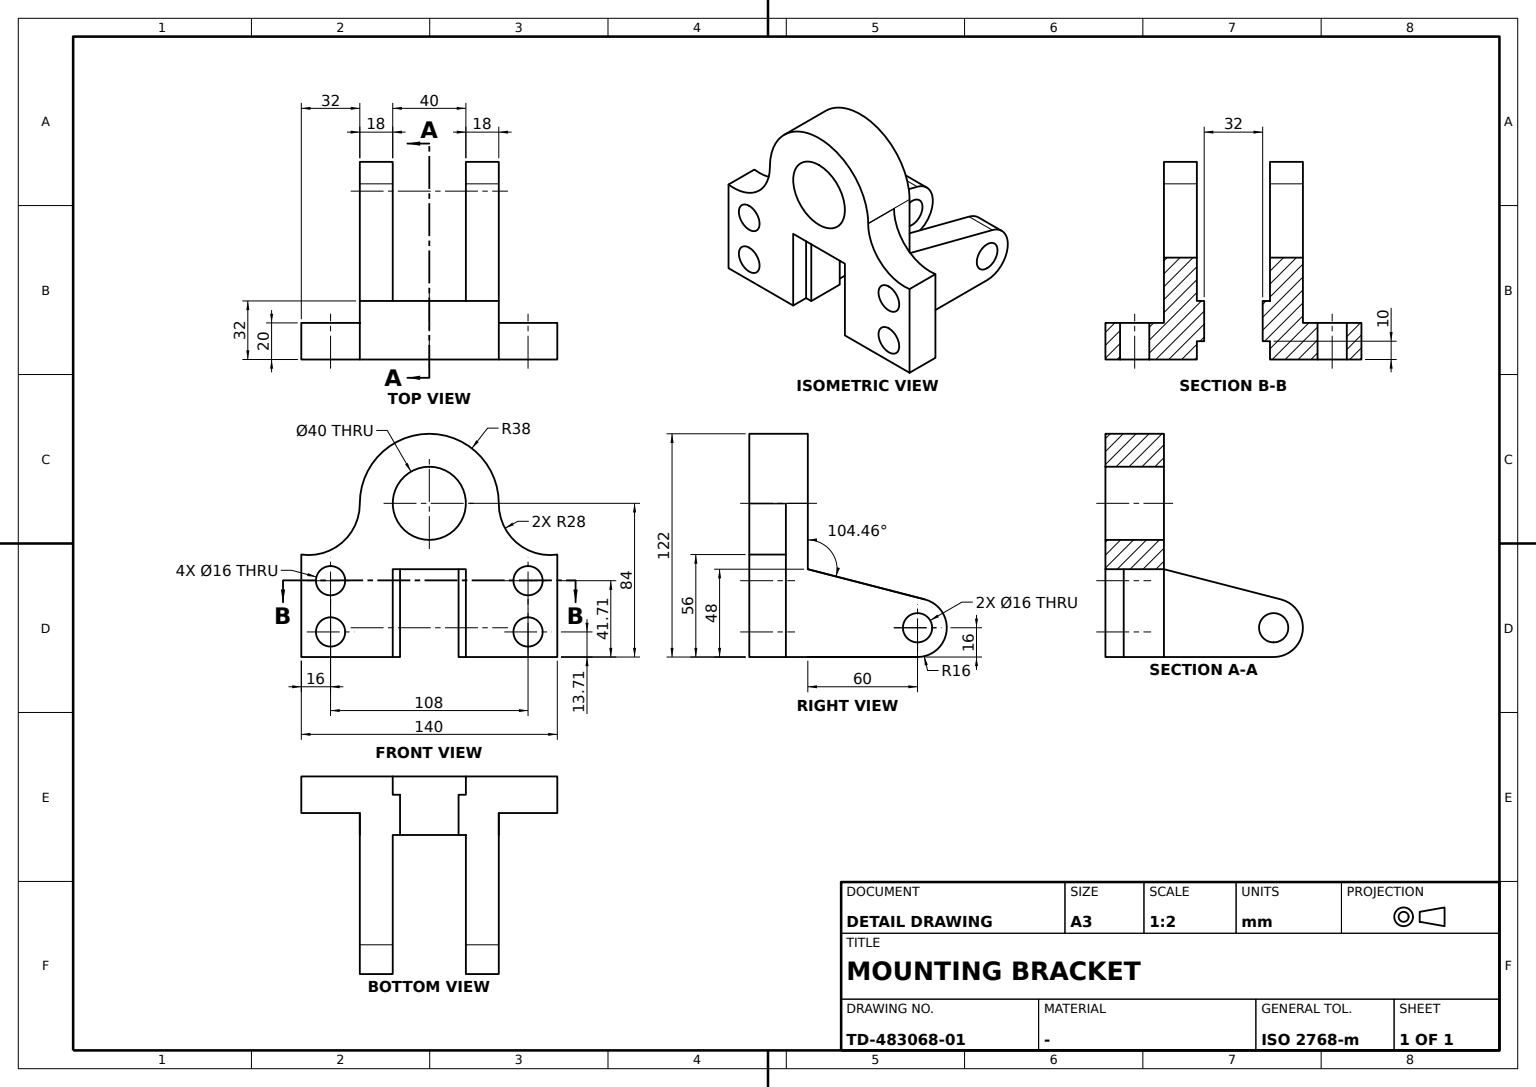
ISO-10303-21;
HEADER;
FILE_DESCRIPTION((''),'2;1');
FILE_NAME('','',(''),(''),'','','');
FILE_SCHEMA(('AUTOMOTIVE_DESIGN'));
ENDSEC;
DATA;
#1=APPLICATION_CONTEXT('');
#2=PRODUCT_CONTEXT('',#1,'mechanical');
#3=PRODUCT('','','',(#2));
#4=PRODUCT_DEFINITION_FORMATION('','',#3);
#5=PRODUCT_DEFINITION_CONTEXT('',#1,'design');
#6=PRODUCT_DEFINITION('','',#4,#5);
#7=PRODUCT_DEFINITION_SHAPE('','',#6);
#8=(LENGTH_UNIT()NAMED_UNIT(*)SI_UNIT(.MILLI.,.METRE.));
#9=(NAMED_UNIT(*)PLANE_ANGLE_UNIT()SI_UNIT($,.RADIAN.));
#10=(NAMED_UNIT(*)SI_UNIT($,.STERADIAN.)SOLID_ANGLE_UNIT());
#11=UNCERTAINTY_MEASURE_WITH_UNIT(LENGTH_MEASURE(0.005),#8,'distance_accuracy_value','');
#12=(GEOMETRIC_REPRESENTATION_CONTEXT(3)GLOBAL_UNCERTAINTY_ASSIGNED_CONTEXT((#11))GLOBAL_UNIT_ASSIGNED_CONTEXT((#8,#9,#10))REPRESENTATION_CONTEXT('',''));
#13=CARTESIAN_POINT('',(-16.,32.,-84.));
#14=VERTEX_POINT('',#13);
#15=CARTESIAN_POINT('',(-16.,10.,-84.));
#16=VERTEX_POINT('',#15);
#17=CARTESIAN_POINT('',(-16.,0.,-84.));
#18=DIRECTION('',(0.,-1.,0.));
#19=VECTOR('',#18,1000.);
#20=LINE('',#17,#19);
#21=EDGE_CURVE('',#14,#16,#20,.T.);
#22=ORIENTED_EDGE('',*,*,#21,.T.);
#23=CARTESIAN_POINT('',(-20.,10.,-84.));
#24=VERTEX_POINT('',#23);
#25=CARTESIAN_POINT('',(0.,10.,-84.));
#26=DIRECTION('',(-1.,0.,0.));
#27=VECTOR('',#26,1000.);
#28=LINE('',#25,#27);
#29=EDGE_CURVE('',#16,#24,#28,.T.);
#30=ORIENTED_EDGE('',*,*,#29,.T.);
#31=CARTESIAN_POINT('',(-20.,0.,-84.));
#32=VERTEX_POINT('',#31);
#33=CARTESIAN_POINT('',(-20.,32.,-84.));
#34=DIRECTION('',(0.,1.,0.));
#35=VECTOR('',#34,1000.);
#36=LINE('',#33,#35);
#37=EDGE_CURVE('',#32,#24,#36,.T.);
#38=ORIENTED_EDGE('',*,*,#37,.F.);
#39=CARTESIAN_POINT('',(-70.,0.,-84.));
#40=VERTEX_POINT('',#39);
#41=CARTESIAN_POINT('',(0.,0.,-84.));
#42=LINE('',#41,#27);
#43=EDGE_CURVE('',#32,#40,#42,.T.);
#44=ORIENTED_EDGE('',*,*,#43,.T.);
#45=CARTESIAN_POINT('',(-70.,20.,-84.));
#46=VERTEX_POINT('',#45);
#47=LINE('',#39,#35);
#48=EDGE_CURVE('',#40,#46,#47,.T.);
#49=ORIENTED_EDGE('',*,*,#48,.T.);
#50=CARTESIAN_POINT('',(-38.,20.,-84.));
#51=VERTEX_POINT('',#50);
#52=CARTESIAN_POINT('',(0.,20.,-84.));
#53=LINE('',#52,#27);
#54=EDGE_CURVE('',#51,#46,#53,.T.);
#55=ORIENTED_EDGE('',*,*,#54,.F.);
#56=CARTESIAN_POINT('',(-38.,92.,-84.));
#57=VERTEX_POINT('',#56);
#58=CARTESIAN_POINT('',(-38.,0.,-84.));
#59=LINE('',#58,#35);
#60=EDGE_CURVE('',#51,#57,#59,.T.);
#61=ORIENTED_EDGE('',*,*,#60,.T.);
#62=CARTESIAN_POINT('',(-20.,92.,-84.));
#63=VERTEX_POINT('',#62);
#64=CARTESIAN_POINT('',(-29.,92.,-84.));
#65=DIRECTION('',(1.,0.,0.));
#66=VECTOR('',#65,1000.);
#67=LINE('',#64,#66);
#68=EDGE_CURVE('',#63,#57,#67,.F.);
#69=ORIENTED_EDGE('',*,*,#68,.F.);
#70=VERTEX_POINT('',#33);
#71=EDGE_CURVE('',#70,#63,#36,.T.);
#72=ORIENTED_EDGE('',*,*,#71,.F.);
#73=CARTESIAN_POINT('',(0.,32.,-84.));
#74=LINE('',#73,#27);
#75=EDGE_CURVE('',#14,#70,#74,.T.);
#76=ORIENTED_EDGE('',*,*,#75,.F.);
#77=EDGE_LOOP('',(#22,#30,#38,#44,#49,#55,#61,#69,#72,#76));
#78=FACE_BOUND('',#77,.T.);
#79=CARTESIAN_POINT('',(38.,0.,-84.));
#80=DIRECTION('',(0.,0.,-1.));
#81=AXIS2_PLACEMENT_3D('',#79,#80,#26);
#82=PLANE('',#81);
#83=ADVANCED_FACE('',(#78),#82,.T.);
#84=CARTESIAN_POINT('',(38.,20.,-84.));
#85=VERTEX_POINT('',#84);
#86=CARTESIAN_POINT('',(70.,20.,-84.));
#87=VERTEX_POINT('',#86);
#88=LINE('',#84,#66);
#89=EDGE_CURVE('',#85,#87,#88,.T.);
#90=ORIENTED_EDGE('',*,*,#89,.F.);
#91=CARTESIAN_POINT('',(38.,20.,-0.287187));
#92=VERTEX_POINT('',#91);
#93=CARTESIAN_POINT('',(38.,20.,0.));
#94=DIRECTION('',(0.,0.,1.));
#95=VECTOR('',#94,1000.);
#96=LINE('',#93,#95);
#97=EDGE_CURVE('',#85,#92,#96,.T.);
#98=ORIENTED_EDGE('',*,*,#97,.T.);
#99=CARTESIAN_POINT('',(70.,20.,-28.));
#100=VERTEX_POINT('',#99);
#101=CARTESIAN_POINT('',(66.,20.,-0.287187));
#102=AXIS2_PLACEMENT_3D('',#101,#34,#94);
#103=CIRCLE('',#102,28.);
#104=EDGE_CURVE('',#100,#92,#103,.T.);
#105=ORIENTED_EDGE('',*,*,#104,.F.);
#106=CARTESIAN_POINT('',(70.,20.,0.));
#107=LINE('',#106,#95);
#108=EDGE_CURVE('',#87,#100,#107,.T.);
#109=ORIENTED_EDGE('',*,*,#108,.F.);
#110=EDGE_LOOP('',(#90,#98,#105,#109));
#111=FACE_BOUND('',#110,.T.);
#112=CARTESIAN_POINT('',(54.,20.,-34.287187));
#113=VERTEX_POINT('',#112);
#114=CARTESIAN_POINT('',(54.,20.,-42.287187));
#115=AXIS2_PLACEMENT_3D('',#114,#34,#94);
#116=CIRCLE('',#115,8.);
#117=EDGE_CURVE('',#113,#113,#116,.T.);
#118=ORIENTED_EDGE('',*,*,#117,.F.);
#119=EDGE_LOOP('',(#118));
#120=FACE_BOUND('',#119,.T.);
#121=CARTESIAN_POINT('',(54.,20.,-62.287187));
#122=VERTEX_POINT('',#121);
#123=CARTESIAN_POINT('',(54.,20.,-70.287187));
#124=AXIS2_PLACEMENT_3D('',#123,#34,#94);
#125=CIRCLE('',#124,8.);
#126=EDGE_CURVE('',#122,#122,#125,.T.);
#127=ORIENTED_EDGE('',*,*,#126,.F.);
#128=EDGE_LOOP('',(#127));
#129=FACE_BOUND('',#128,.T.);
#130=CARTESIAN_POINT('',(0.,20.,0.));
#131=AXIS2_PLACEMENT_3D('',#130,#34,#26);
#132=PLANE('',#131);
#133=ADVANCED_FACE('',(#111,#120,#129),#132,.T.);
#134=ORIENTED_EDGE('',*,*,#37,.T.);
#135=CARTESIAN_POINT('',(-20.,10.,-36.));
#136=VERTEX_POINT('',#135);
#137=CARTESIAN_POINT('',(-20.,10.,0.));
#138=VECTOR('',#80,1000.);
#139=LINE('',#137,#138);
#140=EDGE_CURVE('',#136,#24,#139,.T.);
#141=ORIENTED_EDGE('',*,*,#140,.F.);
#142=CARTESIAN_POINT('',(-20.,0.,-36.));
#143=VERTEX_POINT('',#142);
#144=CARTESIAN_POINT('',(-20.,32.,-36.));
#145=LINE('',#144,#35);
#146=EDGE_CURVE('',#143,#136,#145,.T.);
#147=ORIENTED_EDGE('',*,*,#146,.F.);
#148=LINE('',#31,#95);
#149=EDGE_CURVE('',#32,#143,#148,.T.);
#150=ORIENTED_EDGE('',*,*,#149,.F.);
#151=EDGE_LOOP('',(#134,#141,#147,#150));
#152=FACE_BOUND('',#151,.T.);
#153=AXIS2_PLACEMENT_3D('',#33,#65,#94);
#154=PLANE('',#153);
#155=ADVANCED_FACE('',(#152),#154,.T.);
#156=CARTESIAN_POINT('',(-38.,20.,-0.287187));
#157=VERTEX_POINT('',#156);
#158=CARTESIAN_POINT('',(-70.,20.,-28.));
#159=VERTEX_POINT('',#158);
#160=CARTESIAN_POINT('',(-66.,20.,-0.287187));
#161=AXIS2_PLACEMENT_3D('',#160,#34,#94);
#162=CIRCLE('',#161,28.);
#163=EDGE_CURVE('',#157,#159,#162,.T.);
#164=ORIENTED_EDGE('',*,*,#163,.F.);
#165=CARTESIAN_POINT('',(-38.,20.,0.));
#166=LINE('',#165,#95);
#167=EDGE_CURVE('',#51,#157,#166,.T.);
#168=ORIENTED_EDGE('',*,*,#167,.F.);
#169=ORIENTED_EDGE('',*,*,#54,.T.);
#170=CARTESIAN_POINT('',(-70.,20.,0.));
#171=LINE('',#170,#95);
#172=EDGE_CURVE('',#46,#159,#171,.T.);
#173=ORIENTED_EDGE('',*,*,#172,.T.);
#174=EDGE_LOOP('',(#164,#168,#169,#173));
#175=FACE_BOUND('',#174,.T.);
#176=CARTESIAN_POINT('',(-54.,20.,-62.287187));
#177=VERTEX_POINT('',#176);
#178=CARTESIAN_POINT('',(-54.,20.,-70.287187));
#179=AXIS2_PLACEMENT_3D('',#178,#34,#94);
#180=CIRCLE('',#179,8.);
#181=EDGE_CURVE('',#177,#177,#180,.T.);
#182=ORIENTED_EDGE('',*,*,#181,.F.);
#183=EDGE_LOOP('',(#182));
#184=FACE_BOUND('',#183,.T.);
#185=CARTESIAN_POINT('',(-54.,20.,-34.287187));
#186=VERTEX_POINT('',#185);
#187=CARTESIAN_POINT('',(-54.,20.,-42.287187));
#188=AXIS2_PLACEMENT_3D('',#187,#34,#94);
#189=CIRCLE('',#188,8.);
#190=EDGE_CURVE('',#186,#186,#189,.T.);
#191=ORIENTED_EDGE('',*,*,#190,.F.);
#192=EDGE_LOOP('',(#191));
#193=FACE_BOUND('',#192,.T.);
#194=ADVANCED_FACE('',(#175,#184,#193),#132,.T.);
#195=CARTESIAN_POINT('',(0.,32.,20.));
#196=VERTEX_POINT('',#195);
#197=CARTESIAN_POINT('',(0.,32.,0.));
#198=AXIS2_PLACEMENT_3D('',#197,#34,#94);
#199=CIRCLE('',#198,20.);
#200=EDGE_CURVE('',#196,#196,#199,.T.);
#201=ORIENTED_EDGE('',*,*,#200,.F.);
#202=EDGE_LOOP('',(#201));
#203=FACE_BOUND('',#202,.T.);
#204=CARTESIAN_POINT('',(16.,32.,-84.));
#205=VERTEX_POINT('',#204);
#206=CARTESIAN_POINT('',(16.,32.,-36.));
#207=VERTEX_POINT('',#206);
#208=LINE('',#204,#95);
#209=EDGE_CURVE('',#205,#207,#208,.T.);
#210=ORIENTED_EDGE('',*,*,#209,.T.);
#211=CARTESIAN_POINT('',(-16.,32.,-36.));
#212=VERTEX_POINT('',#211);
#213=CARTESIAN_POINT('',(20.,32.,-36.));
#214=LINE('',#213,#27);
#215=EDGE_CURVE('',#207,#212,#214,.T.);
#216=ORIENTED_EDGE('',*,*,#215,.T.);
#217=LINE('',#13,#95);
#218=EDGE_CURVE('',#14,#212,#217,.T.);
#219=ORIENTED_EDGE('',*,*,#218,.F.);
#220=ORIENTED_EDGE('',*,*,#75,.T.);
#221=VERTEX_POINT('',#144);
#222=CARTESIAN_POINT('',(-20.,32.,0.));
#223=LINE('',#222,#138);
#224=EDGE_CURVE('',#221,#70,#223,.T.);
#225=ORIENTED_EDGE('',*,*,#224,.F.);
#226=CARTESIAN_POINT('',(-38.,32.,-36.));
#227=VERTEX_POINT('',#226);
#228=LINE('',#144,#27);
#229=EDGE_CURVE('',#221,#227,#228,.T.);
#230=ORIENTED_EDGE('',*,*,#229,.T.);
#231=CARTESIAN_POINT('',(-38.,32.,0.));
#232=VERTEX_POINT('',#231);
#233=LINE('',#231,#95);
#234=EDGE_CURVE('',#227,#232,#233,.T.);
#235=ORIENTED_EDGE('',*,*,#234,.T.);
#236=CARTESIAN_POINT('',(38.,32.,0.));
#237=VERTEX_POINT('',#236);
#238=CIRCLE('',#198,38.);
#239=EDGE_CURVE('',#232,#237,#238,.T.);
#240=ORIENTED_EDGE('',*,*,#239,.T.);
#241=CARTESIAN_POINT('',(38.,32.,-36.));
#242=VERTEX_POINT('',#241);
#243=LINE('',#236,#138);
#244=EDGE_CURVE('',#237,#242,#243,.T.);
#245=ORIENTED_EDGE('',*,*,#244,.T.);
#246=VERTEX_POINT('',#213);
#247=EDGE_CURVE('',#242,#246,#228,.T.);
#248=ORIENTED_EDGE('',*,*,#247,.T.);
#249=CARTESIAN_POINT('',(20.,32.,-84.));
#250=VERTEX_POINT('',#249);
#251=LINE('',#213,#138);
#252=EDGE_CURVE('',#246,#250,#251,.T.);
#253=ORIENTED_EDGE('',*,*,#252,.T.);
#254=CARTESIAN_POINT('',(38.,32.,-84.));
#255=LINE('',#254,#66);
#256=EDGE_CURVE('',#205,#250,#255,.T.);
#257=ORIENTED_EDGE('',*,*,#256,.F.);
#258=EDGE_LOOP('',(#210,#216,#219,#220,#225,#230,#235,#240,#245,#248,#253,#257));
#259=FACE_BOUND('',#258,.T.);
#260=AXIS2_PLACEMENT_3D('',#197,#34,#26);
#261=PLANE('',#260);
#262=ADVANCED_FACE('',(#203,#259),#261,.T.);
#263=CARTESIAN_POINT('',(70.,0.,-28.));
#264=VERTEX_POINT('',#263);
#265=CARTESIAN_POINT('',(38.,0.,-0.287187));
#266=VERTEX_POINT('',#265);
#267=CARTESIAN_POINT('',(66.,0.,-0.287187));
#268=AXIS2_PLACEMENT_3D('',#267,#34,#94);
#269=CIRCLE('',#268,28.);
#270=EDGE_CURVE('',#264,#266,#269,.T.);
#271=ORIENTED_EDGE('',*,*,#270,.F.);
#272=LINE('',#263,#35);
#273=EDGE_CURVE('',#264,#100,#272,.T.);
#274=ORIENTED_EDGE('',*,*,#273,.T.);
#275=ORIENTED_EDGE('',*,*,#104,.T.);
#276=CARTESIAN_POINT('',(38.,10.,-0.287187));
#277=LINE('',#276,#35);
#278=EDGE_CURVE('',#266,#92,#277,.T.);
#279=ORIENTED_EDGE('',*,*,#278,.F.);
#280=EDGE_LOOP('',(#271,#274,#275,#279));
#281=FACE_BOUND('',#280,.T.);
#282=CARTESIAN_POINT('',(66.,10.,-0.287187));
#283=AXIS2_PLACEMENT_3D('',#282,#34,#26);
#284=CYLINDRICAL_SURFACE('',#283,28.);
#285=ADVANCED_FACE('',(#281),#284,.F.);
#286=CARTESIAN_POINT('',(38.,92.,-76.));
#287=VERTEX_POINT('',#286);
#288=CARTESIAN_POINT('',(38.,92.,-68.));
#289=AXIS2_PLACEMENT_3D('',#288,#65,#80);
#290=CIRCLE('',#289,8.);
#291=EDGE_CURVE('',#287,#287,#290,.T.);
#292=ORIENTED_EDGE('',*,*,#291,.F.);
#293=EDGE_LOOP('',(#292));
#294=FACE_BOUND('',#293,.T.);
#295=ORIENTED_EDGE('',*,*,#278,.T.);
#296=ORIENTED_EDGE('',*,*,#97,.F.);
#297=CARTESIAN_POINT('',(38.,92.,-84.));
#298=VERTEX_POINT('',#297);
#299=LINE('',#79,#35);
#300=EDGE_CURVE('',#85,#298,#299,.T.);
#301=ORIENTED_EDGE('',*,*,#300,.T.);
#302=CARTESIAN_POINT('',(38.,95.996218,-52.507091));
#303=VERTEX_POINT('',#302);
#304=CIRCLE('',#289,16.);
#305=EDGE_CURVE('',#298,#303,#304,.T.);
#306=ORIENTED_EDGE('',*,*,#305,.T.);
#307=DIRECTION('',(0.,0.968306833,-0.249763644));
#308=VECTOR('',#307,1000.);
#309=LINE('',#241,#308);
#310=EDGE_CURVE('',#242,#303,#309,.T.);
#311=ORIENTED_EDGE('',*,*,#310,.F.);
#312=ORIENTED_EDGE('',*,*,#244,.F.);
#313=CARTESIAN_POINT('',(38.,0.,0.));
#314=VERTEX_POINT('',#313);
#315=CARTESIAN_POINT('',(38.,16.,0.));
#316=LINE('',#315,#35);
#317=EDGE_CURVE('',#314,#237,#316,.T.);
#318=ORIENTED_EDGE('',*,*,#317,.F.);
#319=LINE('',#313,#138);
#320=EDGE_CURVE('',#314,#266,#319,.T.);
#321=ORIENTED_EDGE('',*,*,#320,.T.);
#322=EDGE_LOOP('',(#295,#296,#301,#306,#311,#312,#318,#321));
#323=FACE_BOUND('',#322,.T.);
#324=AXIS2_PLACEMENT_3D('',#313,#65,#80);
#325=PLANE('',#324);
#326=ADVANCED_FACE('',(#294,#323),#325,.T.);
#327=CARTESIAN_POINT('',(20.,10.,-36.));
#328=VERTEX_POINT('',#327);
#329=CARTESIAN_POINT('',(16.,10.,-36.));
#330=VERTEX_POINT('',#329);
#331=LINE('',#327,#27);
#332=EDGE_CURVE('',#328,#330,#331,.T.);
#333=ORIENTED_EDGE('',*,*,#332,.T.);
#334=CARTESIAN_POINT('',(16.,10.,-84.));
#335=VERTEX_POINT('',#334);
#336=LINE('',#334,#95);
#337=EDGE_CURVE('',#335,#330,#336,.T.);
#338=ORIENTED_EDGE('',*,*,#337,.F.);
#339=CARTESIAN_POINT('',(20.,10.,-84.));
#340=VERTEX_POINT('',#339);
#341=CARTESIAN_POINT('',(38.,10.,-84.));
#342=LINE('',#341,#66);
#343=EDGE_CURVE('',#335,#340,#342,.T.);
#344=ORIENTED_EDGE('',*,*,#343,.T.);
#345=LINE('',#327,#138);
#346=EDGE_CURVE('',#328,#340,#345,.T.);
#347=ORIENTED_EDGE('',*,*,#346,.F.);
#348=EDGE_LOOP('',(#333,#338,#344,#347));
#349=FACE_BOUND('',#348,.T.);
#350=CARTESIAN_POINT('',(0.,10.,0.));
#351=AXIS2_PLACEMENT_3D('',#350,#34,#26);
#352=PLANE('',#351);
#353=ADVANCED_FACE('',(#349),#352,.F.);
#354=ORIENTED_EDGE('',*,*,#167,.T.);
#355=CARTESIAN_POINT('',(-38.,0.,-0.287187));
#356=VERTEX_POINT('',#355);
#357=CARTESIAN_POINT('',(-38.,10.,-0.287187));
#358=LINE('',#357,#35);
#359=EDGE_CURVE('',#356,#157,#358,.T.);
#360=ORIENTED_EDGE('',*,*,#359,.F.);
#361=CARTESIAN_POINT('',(-38.,0.,0.));
#362=VERTEX_POINT('',#361);
#363=LINE('',#361,#95);
#364=EDGE_CURVE('',#356,#362,#363,.T.);
#365=ORIENTED_EDGE('',*,*,#364,.T.);
#366=CARTESIAN_POINT('',(-38.,16.,0.));
#367=LINE('',#366,#35);
#368=EDGE_CURVE('',#362,#232,#367,.T.);
#369=ORIENTED_EDGE('',*,*,#368,.T.);
#370=ORIENTED_EDGE('',*,*,#234,.F.);
#371=CARTESIAN_POINT('',(-38.,95.996218,-52.507091));
#372=VERTEX_POINT('',#371);
#373=CARTESIAN_POINT('',(-38.,13.604917,-31.255199));
#374=LINE('',#373,#308);
#375=EDGE_CURVE('',#227,#372,#374,.T.);
#376=ORIENTED_EDGE('',*,*,#375,.T.);
#377=CARTESIAN_POINT('',(-38.,92.,-68.));
#378=AXIS2_PLACEMENT_3D('',#377,#26,#94);
#379=CIRCLE('',#378,16.);
#380=EDGE_CURVE('',#57,#372,#379,.F.);
#381=ORIENTED_EDGE('',*,*,#380,.F.);
#382=ORIENTED_EDGE('',*,*,#60,.F.);
#383=EDGE_LOOP('',(#354,#360,#365,#369,#370,#376,#381,#382));
#384=FACE_BOUND('',#383,.T.);
#385=CARTESIAN_POINT('',(-38.,92.,-60.));
#386=VERTEX_POINT('',#385);
#387=CIRCLE('',#378,8.);
#388=EDGE_CURVE('',#386,#386,#387,.T.);
#389=ORIENTED_EDGE('',*,*,#388,.F.);
#390=EDGE_LOOP('',(#389));
#391=FACE_BOUND('',#390,.T.);
#392=AXIS2_PLACEMENT_3D('',#58,#26,#94);
#393=PLANE('',#392);
#394=ADVANCED_FACE('',(#384,#391),#393,.T.);
#395=ORIENTED_EDGE('',*,*,#48,.F.);
#396=CARTESIAN_POINT('',(-70.,0.,-28.));
#397=VERTEX_POINT('',#396);
#398=CARTESIAN_POINT('',(-70.,0.,0.));
#399=LINE('',#398,#95);
#400=EDGE_CURVE('',#40,#397,#399,.T.);
#401=ORIENTED_EDGE('',*,*,#400,.T.);
#402=LINE('',#396,#35);
#403=EDGE_CURVE('',#397,#159,#402,.T.);
#404=ORIENTED_EDGE('',*,*,#403,.T.);
#405=ORIENTED_EDGE('',*,*,#172,.F.);
#406=EDGE_LOOP('',(#395,#401,#404,#405));
#407=FACE_BOUND('',#406,.T.);
#408=AXIS2_PLACEMENT_3D('',#39,#26,#94);
#409=PLANE('',#408);
#410=ADVANCED_FACE('',(#407),#409,.T.);
#411=ORIENTED_EDGE('',*,*,#291,.T.);
#412=EDGE_LOOP('',(#411));
#413=FACE_BOUND('',#412,.T.);
#414=CARTESIAN_POINT('',(20.,92.,-60.));
#415=VERTEX_POINT('',#414);
#416=CARTESIAN_POINT('',(20.,92.,-68.));
#417=AXIS2_PLACEMENT_3D('',#416,#26,#94);
#418=CIRCLE('',#417,8.);
#419=EDGE_CURVE('',#415,#415,#418,.T.);
#420=ORIENTED_EDGE('',*,*,#419,.T.);
#421=EDGE_LOOP('',(#420));
#422=FACE_BOUND('',#421,.T.);
#423=CARTESIAN_POINT('',(-45.66,92.,-68.));
#424=AXIS2_PLACEMENT_3D('',#423,#65,#34);
#425=CYLINDRICAL_SURFACE('',#424,8.);
#426=ADVANCED_FACE('',(#413,#422),#425,.F.);
#427=CARTESIAN_POINT('',(-20.,92.,-76.));
#428=VERTEX_POINT('',#427);
#429=CARTESIAN_POINT('',(-20.,92.,-68.));
#430=AXIS2_PLACEMENT_3D('',#429,#65,#80);
#431=CIRCLE('',#430,8.);
#432=EDGE_CURVE('',#428,#428,#431,.T.);
#433=ORIENTED_EDGE('',*,*,#432,.F.);
#434=EDGE_LOOP('',(#433));
#435=FACE_BOUND('',#434,.T.);
#436=ORIENTED_EDGE('',*,*,#224,.T.);
#437=ORIENTED_EDGE('',*,*,#71,.T.);
#438=CARTESIAN_POINT('',(-20.,95.996218,-52.507091));
#439=VERTEX_POINT('',#438);
#440=CIRCLE('',#430,16.);
#441=EDGE_CURVE('',#63,#439,#440,.T.);
#442=ORIENTED_EDGE('',*,*,#441,.T.);
#443=LINE('',#144,#308);
#444=EDGE_CURVE('',#221,#439,#443,.T.);
#445=ORIENTED_EDGE('',*,*,#444,.F.);
#446=EDGE_LOOP('',(#436,#437,#442,#445));
#447=FACE_BOUND('',#446,.T.);
#448=ADVANCED_FACE('',(#435,#447),#154,.T.);
#449=ORIENTED_EDGE('',*,*,#346,.T.);
#450=CARTESIAN_POINT('',(20.,0.,-84.));
#451=VERTEX_POINT('',#450);
#452=LINE('',#450,#35);
#453=EDGE_CURVE('',#451,#340,#452,.T.);
#454=ORIENTED_EDGE('',*,*,#453,.F.);
#455=CARTESIAN_POINT('',(20.,0.,-36.));
#456=VERTEX_POINT('',#455);
#457=CARTESIAN_POINT('',(20.,0.,0.));
#458=LINE('',#457,#95);
#459=EDGE_CURVE('',#451,#456,#458,.T.);
#460=ORIENTED_EDGE('',*,*,#459,.T.);
#461=LINE('',#213,#35);
#462=EDGE_CURVE('',#456,#328,#461,.T.);
#463=ORIENTED_EDGE('',*,*,#462,.T.);
#464=EDGE_LOOP('',(#449,#454,#460,#463));
#465=FACE_BOUND('',#464,.T.);
#466=AXIS2_PLACEMENT_3D('',#213,#26,#80);
#467=PLANE('',#466);
#468=ADVANCED_FACE('',(#465),#467,.T.);
#469=CARTESIAN_POINT('',(-29.,95.996218,-52.507091));
#470=LINE('',#469,#66);
#471=EDGE_CURVE('',#439,#372,#470,.F.);
#472=ORIENTED_EDGE('',*,*,#471,.F.);
#473=ORIENTED_EDGE('',*,*,#441,.F.);
#474=ORIENTED_EDGE('',*,*,#68,.T.);
#475=ORIENTED_EDGE('',*,*,#380,.T.);
#476=EDGE_LOOP('',(#472,#473,#474,#475));
#477=FACE_BOUND('',#476,.T.);
#478=CARTESIAN_POINT('',(-29.,92.,-68.));
#479=AXIS2_PLACEMENT_3D('',#478,#65,#34);
#480=CYLINDRICAL_SURFACE('',#479,16.);
#481=ADVANCED_FACE('',(#477),#480,.T.);
#482=ORIENTED_EDGE('',*,*,#29,.F.);
#483=CARTESIAN_POINT('',(-16.,10.,-36.));
#484=VERTEX_POINT('',#483);
#485=LINE('',#15,#95);
#486=EDGE_CURVE('',#16,#484,#485,.T.);
#487=ORIENTED_EDGE('',*,*,#486,.T.);
#488=CARTESIAN_POINT('',(0.,10.,-36.));
#489=LINE('',#488,#66);
#490=EDGE_CURVE('',#484,#136,#489,.F.);
#491=ORIENTED_EDGE('',*,*,#490,.T.);
#492=ORIENTED_EDGE('',*,*,#140,.T.);
#493=EDGE_LOOP('',(#482,#487,#491,#492));
#494=FACE_BOUND('',#493,.T.);
#495=ADVANCED_FACE('',(#494),#352,.F.);
#496=ORIENTED_EDGE('',*,*,#310,.T.);
#497=CARTESIAN_POINT('',(20.,95.996218,-52.507091));
#498=VERTEX_POINT('',#497);
#499=EDGE_CURVE('',#498,#303,#470,.T.);
#500=ORIENTED_EDGE('',*,*,#499,.F.);
#501=LINE('',#213,#308);
#502=EDGE_CURVE('',#246,#498,#501,.T.);
#503=ORIENTED_EDGE('',*,*,#502,.F.);
#504=ORIENTED_EDGE('',*,*,#247,.F.);
#505=EDGE_LOOP('',(#496,#500,#503,#504));
#506=FACE_BOUND('',#505,.T.);
#507=DIRECTION('',(0.,0.249763644,0.968306833));
#508=AXIS2_PLACEMENT_3D('',#144,#507,#307);
#509=PLANE('',#508);
#510=ADVANCED_FACE('',(#506),#509,.T.);
#511=ORIENTED_EDGE('',*,*,#200,.T.);
#512=EDGE_LOOP('',(#511));
#513=FACE_BOUND('',#512,.T.);
#514=CARTESIAN_POINT('',(0.,0.,20.));
#515=VERTEX_POINT('',#514);
#516=CARTESIAN_POINT('',(0.,0.,0.));
#517=AXIS2_PLACEMENT_3D('',#516,#34,#94);
#518=CIRCLE('',#517,20.);
#519=EDGE_CURVE('',#515,#515,#518,.T.);
#520=ORIENTED_EDGE('',*,*,#519,.F.);
#521=EDGE_LOOP('',(#520));
#522=FACE_BOUND('',#521,.T.);
#523=CARTESIAN_POINT('',(0.,16.,0.));
#524=AXIS2_PLACEMENT_3D('',#523,#34,#26);
#525=CYLINDRICAL_SURFACE('',#524,20.);
#526=ADVANCED_FACE('',(#513,#522),#525,.F.);
#527=ORIENTED_EDGE('',*,*,#209,.F.);
#528=CARTESIAN_POINT('',(16.,0.,-84.));
#529=LINE('',#528,#19);
#530=EDGE_CURVE('',#205,#335,#529,.T.);
#531=ORIENTED_EDGE('',*,*,#530,.T.);
#532=ORIENTED_EDGE('',*,*,#337,.T.);
#533=LINE('',#206,#19);
#534=EDGE_CURVE('',#207,#330,#533,.T.);
#535=ORIENTED_EDGE('',*,*,#534,.F.);
#536=EDGE_LOOP('',(#527,#531,#532,#535));
#537=FACE_BOUND('',#536,.T.);
#538=AXIS2_PLACEMENT_3D('',#204,#65,#94);
#539=PLANE('',#538);
#540=ADVANCED_FACE('',(#537),#539,.F.);
#541=ORIENTED_EDGE('',*,*,#388,.T.);
#542=EDGE_LOOP('',(#541));
#543=FACE_BOUND('',#542,.T.);
#544=ORIENTED_EDGE('',*,*,#432,.T.);
#545=EDGE_LOOP('',(#544));
#546=FACE_BOUND('',#545,.T.);
#547=ADVANCED_FACE('',(#543,#546),#425,.F.);
#548=ORIENTED_EDGE('',*,*,#519,.T.);
#549=EDGE_LOOP('',(#548));
#550=FACE_BOUND('',#549,.T.);
#551=CARTESIAN_POINT('',(54.,0.,-34.287187));
#552=VERTEX_POINT('',#551);
#553=CARTESIAN_POINT('',(54.,0.,-42.287187));
#554=AXIS2_PLACEMENT_3D('',#553,#34,#94);
#555=CIRCLE('',#554,8.);
#556=EDGE_CURVE('',#552,#552,#555,.T.);
#557=ORIENTED_EDGE('',*,*,#556,.T.);
#558=EDGE_LOOP('',(#557));
#559=FACE_BOUND('',#558,.T.);
#560=CARTESIAN_POINT('',(-54.,0.,-34.287187));
#561=VERTEX_POINT('',#560);
#562=CARTESIAN_POINT('',(-54.,0.,-42.287187));
#563=AXIS2_PLACEMENT_3D('',#562,#34,#94);
#564=CIRCLE('',#563,8.);
#565=EDGE_CURVE('',#561,#561,#564,.T.);
#566=ORIENTED_EDGE('',*,*,#565,.T.);
#567=EDGE_LOOP('',(#566));
#568=FACE_BOUND('',#567,.T.);
#569=CARTESIAN_POINT('',(54.,0.,-62.287187));
#570=VERTEX_POINT('',#569);
#571=CARTESIAN_POINT('',(54.,0.,-70.287187));
#572=AXIS2_PLACEMENT_3D('',#571,#34,#94);
#573=CIRCLE('',#572,8.);
#574=EDGE_CURVE('',#570,#570,#573,.T.);
#575=ORIENTED_EDGE('',*,*,#574,.T.);
#576=EDGE_LOOP('',(#575));
#577=FACE_BOUND('',#576,.T.);
#578=CARTESIAN_POINT('',(-54.,0.,-62.287187));
#579=VERTEX_POINT('',#578);
#580=CARTESIAN_POINT('',(-54.,0.,-70.287187));
#581=AXIS2_PLACEMENT_3D('',#580,#34,#94);
#582=CIRCLE('',#581,8.);
#583=EDGE_CURVE('',#579,#579,#582,.T.);
#584=ORIENTED_EDGE('',*,*,#583,.T.);
#585=EDGE_LOOP('',(#584));
#586=FACE_BOUND('',#585,.T.);
#587=CARTESIAN_POINT('',(-66.,0.,-0.287187));
#588=AXIS2_PLACEMENT_3D('',#587,#34,#94);
#589=CIRCLE('',#588,28.);
#590=EDGE_CURVE('',#356,#397,#589,.T.);
#591=ORIENTED_EDGE('',*,*,#590,.T.);
#592=ORIENTED_EDGE('',*,*,#400,.F.);
#593=ORIENTED_EDGE('',*,*,#43,.F.);
#594=ORIENTED_EDGE('',*,*,#149,.T.);
#595=LINE('',#455,#27);
#596=EDGE_CURVE('',#456,#143,#595,.T.);
#597=ORIENTED_EDGE('',*,*,#596,.F.);
#598=ORIENTED_EDGE('',*,*,#459,.F.);
#599=CARTESIAN_POINT('',(70.,0.,-84.));
#600=VERTEX_POINT('',#599);
#601=LINE('',#79,#66);
#602=EDGE_CURVE('',#451,#600,#601,.T.);
#603=ORIENTED_EDGE('',*,*,#602,.T.);
#604=CARTESIAN_POINT('',(70.,0.,0.));
#605=LINE('',#604,#95);
#606=EDGE_CURVE('',#600,#264,#605,.T.);
#607=ORIENTED_EDGE('',*,*,#606,.T.);
#608=ORIENTED_EDGE('',*,*,#270,.T.);
#609=ORIENTED_EDGE('',*,*,#320,.F.);
#610=CIRCLE('',#517,38.);
#611=EDGE_CURVE('',#362,#314,#610,.T.);
#612=ORIENTED_EDGE('',*,*,#611,.F.);
#613=ORIENTED_EDGE('',*,*,#364,.F.);
#614=EDGE_LOOP('',(#591,#592,#593,#594,#597,#598,#603,#607,#608,#609,#612,#613));
#615=FACE_BOUND('',#614,.T.);
#616=AXIS2_PLACEMENT_3D('',#516,#34,#26);
#617=PLANE('',#616);
#618=ADVANCED_FACE('',(#550,#559,#568,#577,#586,#615),#617,.F.);
#619=ORIENTED_EDGE('',*,*,#471,.T.);
#620=ORIENTED_EDGE('',*,*,#375,.F.);
#621=ORIENTED_EDGE('',*,*,#229,.F.);
#622=ORIENTED_EDGE('',*,*,#444,.T.);
#623=EDGE_LOOP('',(#619,#620,#621,#622));
#624=FACE_BOUND('',#623,.T.);
#625=ADVANCED_FACE('',(#624),#509,.T.);
#626=ORIENTED_EDGE('',*,*,#21,.F.);
#627=ORIENTED_EDGE('',*,*,#218,.T.);
#628=LINE('',#211,#19);
#629=EDGE_CURVE('',#212,#484,#628,.T.);
#630=ORIENTED_EDGE('',*,*,#629,.T.);
#631=ORIENTED_EDGE('',*,*,#486,.F.);
#632=EDGE_LOOP('',(#626,#627,#630,#631));
#633=FACE_BOUND('',#632,.T.);
#634=AXIS2_PLACEMENT_3D('',#13,#65,#94);
#635=PLANE('',#634);
#636=ADVANCED_FACE('',(#633),#635,.T.);
#637=ORIENTED_EDGE('',*,*,#502,.T.);
#638=CARTESIAN_POINT('',(20.,92.,-84.));
#639=VERTEX_POINT('',#638);
#640=CIRCLE('',#417,16.);
#641=EDGE_CURVE('',#639,#498,#640,.F.);
#642=ORIENTED_EDGE('',*,*,#641,.F.);
#643=EDGE_CURVE('',#250,#639,#452,.T.);
#644=ORIENTED_EDGE('',*,*,#643,.F.);
#645=ORIENTED_EDGE('',*,*,#252,.F.);
#646=EDGE_LOOP('',(#637,#642,#644,#645));
#647=FACE_BOUND('',#646,.T.);
#648=ORIENTED_EDGE('',*,*,#419,.F.);
#649=EDGE_LOOP('',(#648));
#650=FACE_BOUND('',#649,.T.);
#651=ADVANCED_FACE('',(#647,#650),#467,.T.);
#652=ORIENTED_EDGE('',*,*,#190,.T.);
#653=EDGE_LOOP('',(#652));
#654=FACE_BOUND('',#653,.T.);
#655=ORIENTED_EDGE('',*,*,#565,.F.);
#656=EDGE_LOOP('',(#655));
#657=FACE_BOUND('',#656,.T.);
#658=CARTESIAN_POINT('',(-54.,10.,-42.287187));
#659=AXIS2_PLACEMENT_3D('',#658,#34,#26);
#660=CYLINDRICAL_SURFACE('',#659,8.);
#661=ADVANCED_FACE('',(#654,#657),#660,.F.);
#662=ORIENTED_EDGE('',*,*,#574,.F.);
#663=EDGE_LOOP('',(#662));
#664=FACE_BOUND('',#663,.T.);
#665=ORIENTED_EDGE('',*,*,#126,.T.);
#666=EDGE_LOOP('',(#665));
#667=FACE_BOUND('',#666,.T.);
#668=CARTESIAN_POINT('',(54.,10.,-70.287187));
#669=AXIS2_PLACEMENT_3D('',#668,#34,#26);
#670=CYLINDRICAL_SURFACE('',#669,8.);
#671=ADVANCED_FACE('',(#664,#667),#670,.F.);
#672=ORIENTED_EDGE('',*,*,#534,.T.);
#673=ORIENTED_EDGE('',*,*,#332,.F.);
#674=ORIENTED_EDGE('',*,*,#462,.F.);
#675=ORIENTED_EDGE('',*,*,#596,.T.);
#676=ORIENTED_EDGE('',*,*,#146,.T.);
#677=ORIENTED_EDGE('',*,*,#490,.F.);
#678=ORIENTED_EDGE('',*,*,#629,.F.);
#679=ORIENTED_EDGE('',*,*,#215,.F.);
#680=EDGE_LOOP('',(#672,#673,#674,#675,#676,#677,#678,#679));
#681=FACE_BOUND('',#680,.T.);
#682=AXIS2_PLACEMENT_3D('',#213,#94,#26);
#683=PLANE('',#682);
#684=ADVANCED_FACE('',(#681),#683,.F.);
#685=ORIENTED_EDGE('',*,*,#181,.T.);
#686=EDGE_LOOP('',(#685));
#687=FACE_BOUND('',#686,.T.);
#688=ORIENTED_EDGE('',*,*,#583,.F.);
#689=EDGE_LOOP('',(#688));
#690=FACE_BOUND('',#689,.T.);
#691=CARTESIAN_POINT('',(-54.,10.,-70.287187));
#692=AXIS2_PLACEMENT_3D('',#691,#34,#26);
#693=CYLINDRICAL_SURFACE('',#692,8.);
#694=ADVANCED_FACE('',(#687,#690),#693,.F.);
#695=ORIENTED_EDGE('',*,*,#117,.T.);
#696=EDGE_LOOP('',(#695));
#697=FACE_BOUND('',#696,.T.);
#698=ORIENTED_EDGE('',*,*,#556,.F.);
#699=EDGE_LOOP('',(#698));
#700=FACE_BOUND('',#699,.T.);
#701=CARTESIAN_POINT('',(54.,10.,-42.287187));
#702=AXIS2_PLACEMENT_3D('',#701,#34,#26);
#703=CYLINDRICAL_SURFACE('',#702,8.);
#704=ADVANCED_FACE('',(#697,#700),#703,.F.);
#705=ORIENTED_EDGE('',*,*,#611,.T.);
#706=ORIENTED_EDGE('',*,*,#317,.T.);
#707=ORIENTED_EDGE('',*,*,#239,.F.);
#708=ORIENTED_EDGE('',*,*,#368,.F.);
#709=EDGE_LOOP('',(#705,#706,#707,#708));
#710=FACE_BOUND('',#709,.T.);
#711=CYLINDRICAL_SURFACE('',#524,38.);
#712=ADVANCED_FACE('',(#710),#711,.T.);
#713=ORIENTED_EDGE('',*,*,#273,.F.);
#714=ORIENTED_EDGE('',*,*,#606,.F.);
#715=LINE('',#599,#35);
#716=EDGE_CURVE('',#600,#87,#715,.T.);
#717=ORIENTED_EDGE('',*,*,#716,.T.);
#718=ORIENTED_EDGE('',*,*,#108,.T.);
#719=EDGE_LOOP('',(#713,#714,#717,#718));
#720=FACE_BOUND('',#719,.T.);
#721=AXIS2_PLACEMENT_3D('',#599,#26,#94);
#722=PLANE('',#721);
#723=ADVANCED_FACE('',(#720),#722,.F.);
#724=ORIENTED_EDGE('',*,*,#343,.F.);
#725=ORIENTED_EDGE('',*,*,#530,.F.);
#726=ORIENTED_EDGE('',*,*,#256,.T.);
#727=ORIENTED_EDGE('',*,*,#643,.T.);
#728=EDGE_CURVE('',#639,#298,#67,.T.);
#729=ORIENTED_EDGE('',*,*,#728,.T.);
#730=ORIENTED_EDGE('',*,*,#300,.F.);
#731=ORIENTED_EDGE('',*,*,#89,.T.);
#732=ORIENTED_EDGE('',*,*,#716,.F.);
#733=ORIENTED_EDGE('',*,*,#602,.F.);
#734=ORIENTED_EDGE('',*,*,#453,.T.);
#735=EDGE_LOOP('',(#724,#725,#726,#727,#729,#730,#731,#732,#733,#734));
#736=FACE_BOUND('',#735,.T.);
#737=ADVANCED_FACE('',(#736),#82,.T.);
#738=ORIENTED_EDGE('',*,*,#590,.F.);
#739=ORIENTED_EDGE('',*,*,#359,.T.);
#740=ORIENTED_EDGE('',*,*,#163,.T.);
#741=ORIENTED_EDGE('',*,*,#403,.F.);
#742=EDGE_LOOP('',(#738,#739,#740,#741));
#743=FACE_BOUND('',#742,.T.);
#744=CARTESIAN_POINT('',(-66.,10.,-0.287187));
#745=AXIS2_PLACEMENT_3D('',#744,#34,#26);
#746=CYLINDRICAL_SURFACE('',#745,28.);
#747=ADVANCED_FACE('',(#743),#746,.F.);
#748=ORIENTED_EDGE('',*,*,#641,.T.);
#749=ORIENTED_EDGE('',*,*,#499,.T.);
#750=ORIENTED_EDGE('',*,*,#305,.F.);
#751=ORIENTED_EDGE('',*,*,#728,.F.);
#752=EDGE_LOOP('',(#748,#749,#750,#751));
#753=FACE_BOUND('',#752,.T.);
#754=ADVANCED_FACE('',(#753),#480,.T.);
#755=CLOSED_SHELL('',(#83,#133,#155,#194,#262,#285,#326,#353,#394,#410,#426,#448,#468,#481,#495,#510,#526,#540,#547,#618,#625,#636,#651,#661,#671,#684,#694,#704,#712,#723,#737,#747,#754));
#756=MANIFOLD_SOLID_BREP('',#755);
#757=ADVANCED_BREP_SHAPE_REPRESENTATION('',(#756),#12);
#758=SHAPE_DEFINITION_REPRESENTATION(#7,#757);
ENDSEC;
END-ISO-10303-21;
